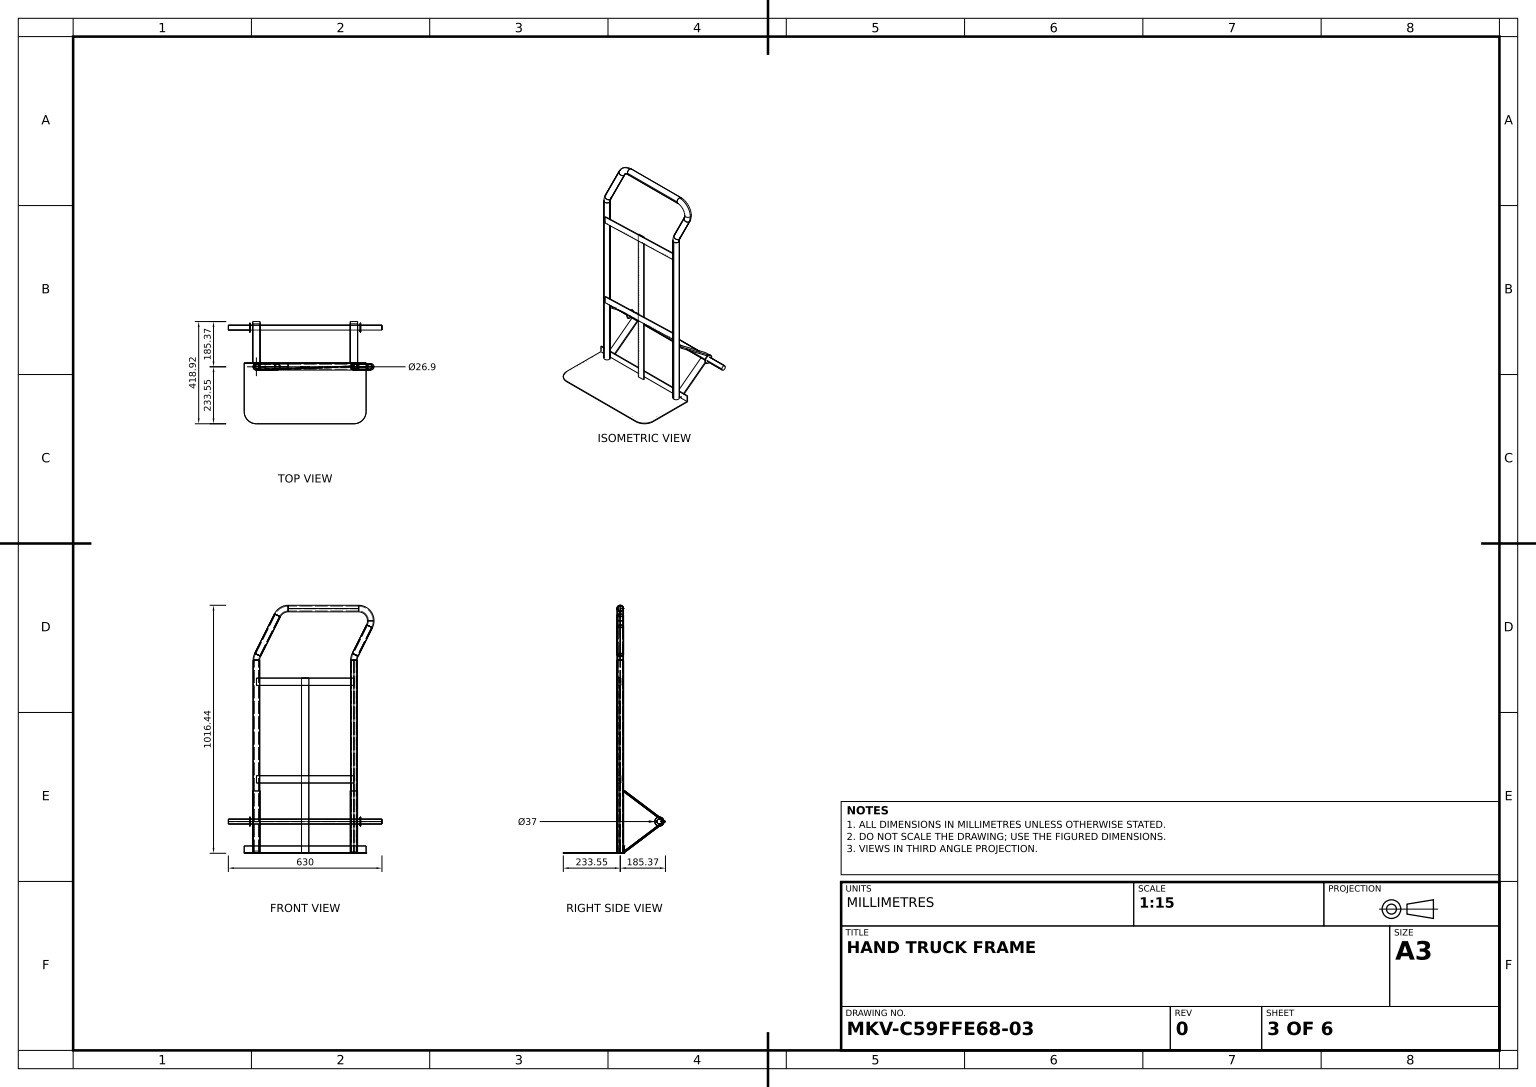
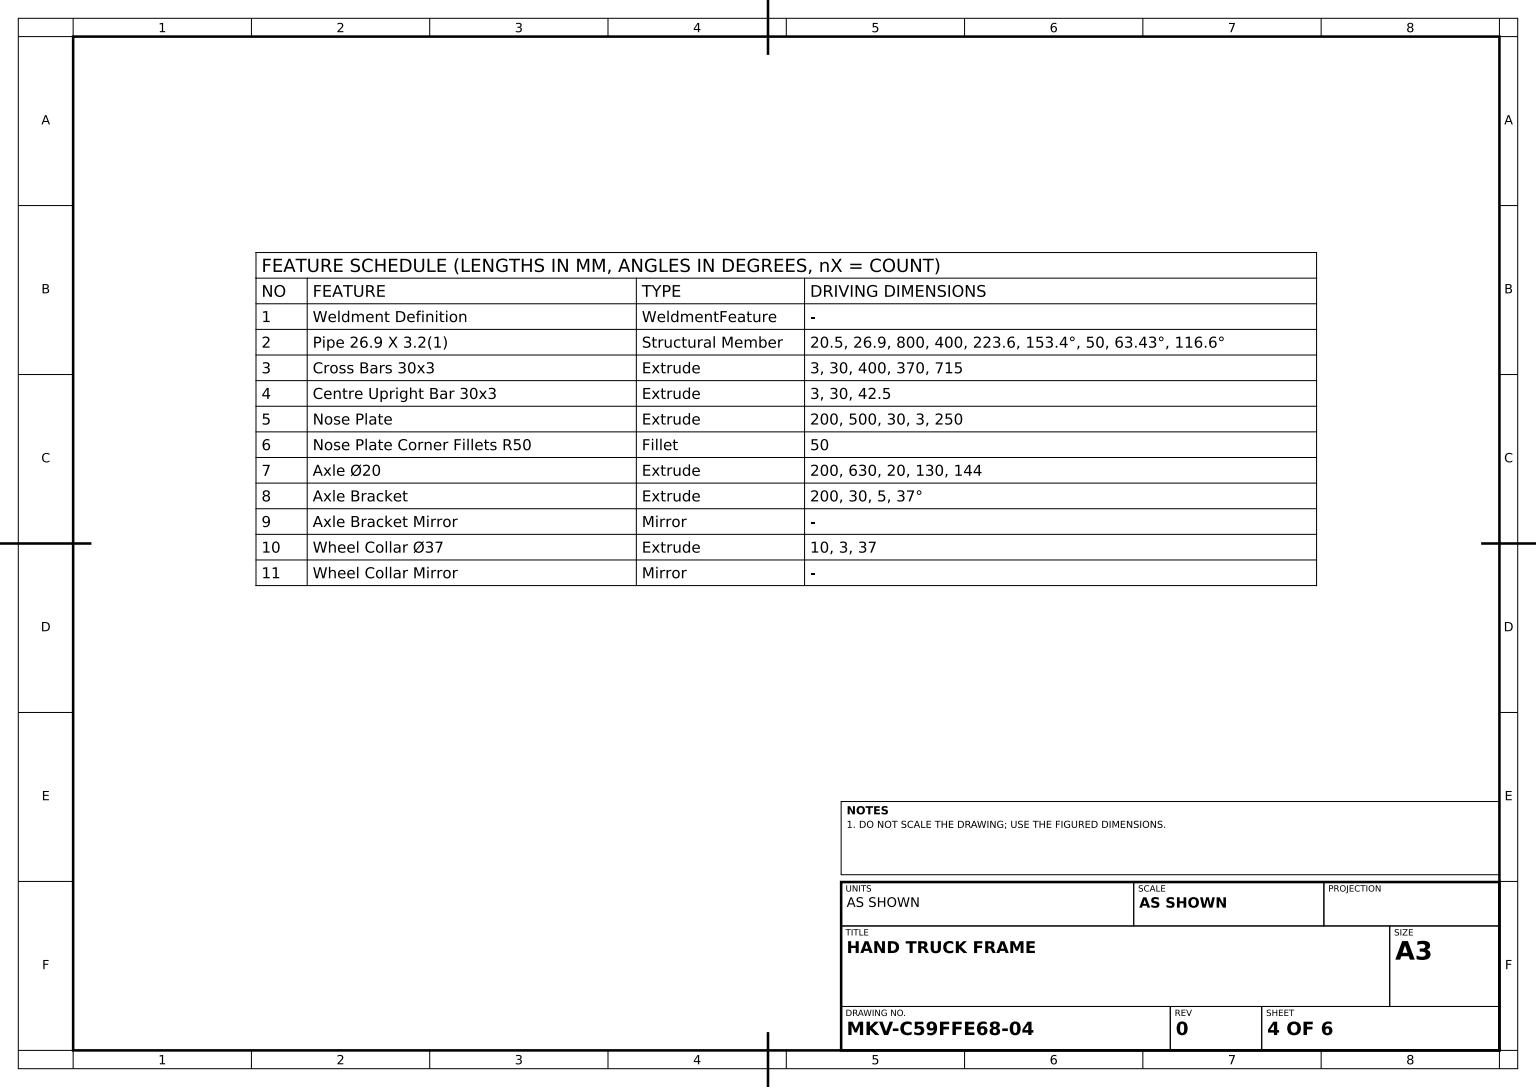
solid
v1 (-406.748954,816.574926,0)
v2 (-413.45,788.194321,0)
e1 v1 v2 CIRCLE(AX(P(-350,788.194321,0),D(0,0,1),D(0,-1,0)),63.45)
v3 (-382.689902,804.542802,0)
e2 v1 v3 CIRCLE(AX(P(-394.719428,810.558864,0),D(-0.447290848,-0.89438856,0),D(-0.89438856,0.447290848,0)),13.45)
v4 (-386.55,788.194321,0)
e3 v3 v4 CIRCLE(AX(P(-350,788.194321,0),D(0,0,1),D(0,-1,0)),36.55)
e4 v4 v2 CIRCLE(AX(P(-400,788.194321,0),D(0,1,0),D(1,0,0)),13.45)
face TORUS(AX(P(-350,788.194321,0),D(0,0,1),D(1,0,0)),50,13.45) [-e1 e2 e3 e4]
e5 v2 v4 CIRCLE(AX(P(-400,788.194321,0),D(0,1,0),D(1,0,0)),13.45)
e6 v3 v1 CIRCLE(AX(P(-394.719428,810.558864,0),D(-0.447290848,-0.89438856,0),D(-0.89438856,0.447290848,0)),13.45)
face TORUS(AX(P(-350,788.194321,0),D(0,0,1),D(1,0,0)),50,13.45) [e5 -e3 e6 e1]
v5 (-403.886911,815.143595,0)
v6 (-385.551945,805.974133,0)
e7 v5 v6 CIRCLE(AX(P(-394.719428,810.558864,0),D(0.447290848,0.89438856,0),D(-0.89438856,0.447290848,0)),10.25)
e8 v6 v5 CIRCLE(AX(P(-394.719428,810.558864,0),D(0.447290848,0.89438856,0),D(-0.89438856,0.447290848,0)),10.25)
face PLANE(AX(P(-394.719428,810.558864,0),D(0.447290848,0.89438856,0),D(-0.89438856,0.447290848,0))) [-e7 -e8] [-e2 -e6]
v7 (-389.75,788.194321,0)
e9 v6 v7 CIRCLE(AX(P(-350,788.194321,0),D(0,0,1),D(0,-1,0)),39.75)
v8 (-410.25,788.194321,0)
e10 v7 v8 CIRCLE(AX(P(-400,788.194321,0),D(0,-1,0),D(1,0,0)),10.25)
e11 v5 v8 CIRCLE(AX(P(-350,788.194321,0),D(0,0,1),D(0,-1,0)),60.25)
face TORUS(AX(P(-350,788.194321,0),D(0,0,1),D(1,0,0)),50,10.25) rev [e9 e10 -e11 e7]
e12 v8 v7 CIRCLE(AX(P(-400,788.194321,0),D(0,-1,0),D(1,0,0)),10.25)
face PLANE(AX(P(-400,788.194321,0),D(0,-1,0),D(1,0,0))) [-e4 -e5] [-e10 -e12]
face TORUS(AX(P(-350,788.194321,0),D(0,0,1),D(1,0,0)),50,10.25) rev [e8 e11 e12 -e9]
solid
v9 (0,788.194321,-13.45)
v10 (0,788.194321,13.45)
e13 v9 v10 CIRCLE(AX(P(0,788.194321,0),D(0,1,0),D(0,0,1)),13.45)
e14 v10 v9 CIRCLE(AX(P(0,788.194321,0),D(0,1,0),D(0,0,1)),13.45)
v11 (0,788.194321,10.25)
v12 (0,788.194321,-10.25)
e15 v11 v12 CIRCLE(AX(P(0,788.194321,0),D(0,1,0),D(0,0,1)),10.25)
e16 v12 v11 CIRCLE(AX(P(0,788.194321,0),D(0,1,0),D(0,0,1)),10.25)
face PLANE(AX(P(0,788.194321,0),D(0,1,0),D(0,0,1))) [e13 e14] [-e15 -e16]
v13 (0,0,10.25)
v14 (0,0,-10.25)
e17 v13 v14 CIRCLE(AX(P(0,0,0),D(0,1,0),D(0,0,1)),10.25)
e18 v11 v13 LINE
e19 v12 v14 LINE
face CYL(AX(P(0,788.194321,0),D(0,-1,0),D(0,0,-1)),10.25) rev [-e17 -e18 e15 e19]
e20 v14 v13 CIRCLE(AX(P(0,0,0),D(0,1,0),D(0,0,1)),10.25)
face CYL(AX(P(0,788.194321,0),D(0,-1,0),D(0,0,-1)),10.25) rev [-e20 -e19 e16 e18]
v15 (0,0,13.45)
v16 (0,0,-13.45)
e21 v15 v16 CIRCLE(AX(P(0,0,0),D(0,1,0),D(0,0,1)),13.45)
e22 v16 v15 CIRCLE(AX(P(0,0,0),D(0,1,0),D(0,0,1)),13.45)
face PLANE(AX(P(0,0,0),D(0,1,0),D(0,0,1))) rev [-e21 -e22] [e17 e20]
e23 v10 v15 LINE
e24 v9 v16 LINE
face CYL(AX(P(0,788.194321,0),D(0,-1,0),D(0,0,-1)),13.45) [e23 e21 -e24 -e14]
face CYL(AX(P(0,788.194321,0),D(0,-1,0),D(0,0,-1)),13.45) [e24 e22 -e23 -e13]
solid
v17 (-304.638996,967.765093,0)
v18 (-322.973962,976.934556,0)
e25 v17 v18 CIRCLE(AX(P(-313.806479,972.349825,0),D(0.447290848,0.89438856,0),D(-0.89438856,0.447290848,0)),10.25)
e26 v18 v17 CIRCLE(AX(P(-313.806479,972.349825,0),D(0.447290848,0.89438856,0),D(-0.89438856,0.447290848,0)),10.25)
v19 (-301.776953,966.333763,0)
v20 (-325.836005,978.365886,0)
e27 v19 v20 CIRCLE(AX(P(-313.806479,972.349825,0),D(0.447290848,0.89438856,0),D(-0.89438856,0.447290848,0)),13.45)
e28 v20 v19 CIRCLE(AX(P(-313.806479,972.349825,0),D(0.447290848,0.89438856,0),D(-0.89438856,0.447290848,0)),13.45)
face PLANE(AX(P(-313.806479,972.349825,0),D(0.447290848,0.89438856,0),D(-0.89438856,0.447290848,0))) [-e25 -e26] [e27 e28]
v21 (-406.748954,816.574926,0)
e29 v21 v20 LINE
v22 (-382.689902,804.542802,0)
e30 v22 v21 CIRCLE(AX(P(-394.719428,810.558864,0),D(-0.447290848,-0.89438856,0),D(0.89438856,-0.447290848,0)),13.45)
e31 v22 v19 LINE
face CYL(AX(P(-394.719428,810.558864,0),D(0.447290848,0.89438856,0),D(-0.89438856,0.447290848,0)),13.45) [-e29 -e30 e31 -e28]
v23 (-385.551945,805.974133,0)
v24 (-403.886911,815.143595,0)
e32 v23 v24 CIRCLE(AX(P(-394.719428,810.558864,0),D(-0.447290848,-0.89438856,0),D(0.89438856,-0.447290848,0)),10.25)
e33 v24 v18 LINE
e34 v23 v17 LINE
face CYL(AX(P(-394.719428,810.558864,0),D(0.447290848,0.89438856,0),D(-0.89438856,0.447290848,0)),10.25) rev [e32 e33 e26 -e34]
e35 v24 v23 CIRCLE(AX(P(-394.719428,810.558864,0),D(-0.447290848,-0.89438856,0),D(0.89438856,-0.447290848,0)),10.25)
e36 v21 v22 CIRCLE(AX(P(-394.719428,810.558864,0),D(-0.447290848,-0.89438856,0),D(0.89438856,-0.447290848,0)),13.45)
face PLANE(AX(P(-394.719428,810.558864,0),D(-0.447290848,-0.89438856,0),D(0.89438856,-0.447290848,0))) [-e35 -e32] [e36 e30]
face CYL(AX(P(-394.719428,810.558864,0),D(0.447290848,0.89438856,0),D(-0.89438856,0.447290848,0)),13.45) [-e27 -e31 -e36 e29]
face CYL(AX(P(-394.719428,810.558864,0),D(0.447290848,0.89438856,0),D(-0.89438856,0.447290848,0)),10.25) rev [-e33 e35 e34 e25]
solid
v25 (0.012157,315,-3.002106)
v26 (-399.761651,315,10.447894)
e37 v25 v26 LINE
v27 (-399.660776,315,13.446197)
e38 v26 v27 LINE
v28 (0.113032,315,-0.003803)
e39 v28 v27 LINE
e40 v25 v28 LINE
face PLANE(AX(P(0.012157,315,-3.002106),D(0,1,0),D(-1,0,0))) [e37 e38 -e39 -e40]
v29 (-399.660776,285,13.446197)
e41 v27 v29 LINE
v30 (0.113032,285,-0.003803)
e42 v29 v30 LINE
e43 v30 v28 LINE
face PLANE(AX(P(0,0,0),D(-0.033625,0,-0.99943452),D(-0.99943452,0,0.033625))) rev [e41 e42 e43 e39]
v31 (-399.761651,285,10.447894)
e44 v31 v29 LINE
v32 (0.012157,285,-3.002106)
e45 v31 v32 LINE
e46 v32 v30 LINE
face PLANE(AX(P(0.012157,285,-3.002106),D(0,-1,0),D(1,0,0))) [-e42 -e44 e45 e46]
e47 v32 v25 LINE
face PLANE(AX(P(0.012157,315,-3.002106),D(0.99943452,0,-0.033625),D(-0.033625,0,-0.99943452))) [e47 e40 -e43 -e46]
e48 v26 v31 LINE
face PLANE(AX(P(-0.100875,0,-2.998304),D(-0.033625,0,-0.99943452),D(-0.99943452,0,0.033625))) [-e45 -e48 -e37 -e47]
face PLANE(AX(P(-399.761651,315,10.447894),D(-0.99943452,0,0.033625),D(0.033625,0,0.99943452))) [-e38 e48 e44 -e41]
solid
v33 (25,127,-178.95)
v34 (25,127,-141.95)
e49 v33 v34 CIRCLE(AX(P(25,127,-160.45),D(1,0,0),D(0,0,-1)),18.5)
e50 v34 v33 CIRCLE(AX(P(25,127,-160.45),D(1,0,0),D(0,0,-1)),18.5)
face PLANE(AX(P(25,127,-160.45),D(1,0,0),D(0,0,-1))) rev [-e49 -e50]
v35 (28,127,-141.95)
v36 (28,127,-178.95)
e51 v35 v36 CIRCLE(AX(P(28,127,-160.45),D(1,0,0),D(0,0,-1)),18.5)
e52 v36 v35 CIRCLE(AX(P(28,127,-160.45),D(1,0,0),D(0,0,-1)),18.5)
face PLANE(AX(P(28,127,-160.45),D(1,0,0),D(0,0,-1))) [e51 e52]
e53 v36 v33 LINE
e54 v35 v34 LINE
face CYL(AX(P(28,127,-160.45),D(-1,0,0),D(0,0,1)),18.5) [-e53 -e51 e54 e50]
face CYL(AX(P(28,127,-160.45),D(-1,0,0),D(0,0,1)),18.5) [-e54 -e52 e53 e49]
solid
v37 (15,250.293802,-13.45)
v38 (-15,250.293802,-13.45)
e55 v37 v38 LINE
v39 (15,254.286979,-16.459075)
e56 v39 v37 LINE
v40 (-15,254.286979,-16.459075)
e57 v39 v40 LINE
e58 v40 v38 LINE
face PLANE(AX(P(15,250.293802,-13.45),D(0,-0.601815023,-0.79863551),D(0,0.79863551,-0.601815023))) rev [-e55 -e56 e57 e58]
v41 (15,127,-177.066401)
e59 v37 v41 LINE
v42 (15,3.706198,-13.45)
e60 v41 v42 LINE
v43 (15,-0.286979,-16.459075)
e61 v42 v43 LINE
v44 (15,127,-185.374602)
e62 v43 v44 LINE
e63 v44 v39 LINE
face PLANE(AX(P(15,0,0),D(1,0,0),D(0,0,-1))) [e59 e60 e61 e62 e63 e56]
v45 (-15,127,-177.066401)
e64 v38 v45 LINE
e65 v41 v45 LINE
face PLANE(AX(P(15,127,-177.066401),D(0,0.79863551,-0.601815023),D(0,0.601815023,0.79863551))) rev [-e59 e55 e64 -e65]
v46 (-15,3.706198,-13.45)
e66 v42 v46 LINE
v47 (-15,-0.286979,-16.459075)
e67 v46 v47 LINE
e68 v43 v47 LINE
face PLANE(AX(P(15,3.706198,-13.45),D(0,0.601815023,-0.79863551),D(0,0.79863551,0.601815023))) rev [-e61 e66 e67 -e68]
v48 (-15,127,-185.374602)
e69 v44 v48 LINE
e70 v48 v40 LINE
face PLANE(AX(P(15,127,-185.374602),D(0,-0.79863551,0.601815023),D(0,-0.601815023,-0.79863551))) rev [-e63 e69 e70 -e57]
e71 v45 v46 LINE
face PLANE(AX(P(15,127,-177.066401),D(0,-0.79863551,-0.601815023),D(0,0.601815023,-0.79863551))) rev [-e66 -e60 e65 e71]
e72 v47 v48 LINE
face PLANE(AX(P(15,127,-185.374602),D(0,0.79863551,0.601815023),D(0,-0.601815023,0.79863551))) rev [e68 e72 -e69 -e62]
face PLANE(AX(P(-15,0,0),D(1,0,0),D(0,0,-1))) rev [-e67 -e71 -e64 -e58 -e70 -e72]
solid
v49 (-184.984104,0,0.220215)
v50 (-214.96714,0,1.228965)
e73 v49 v50 LINE
v51 (-214.96714,715,1.228965)
e74 v50 v51 LINE
v52 (-184.984104,715,0.220215)
e75 v51 v52 LINE
e76 v52 v49 LINE
face PLANE(AX(P(-0.20175,0,-5.996607),D(0.033625,0,0.99943452),D(0.99943452,0,-0.033625))) rev [e73 e74 e75 e76]
v53 (-214.866265,0,4.227269)
e77 v50 v53 LINE
v54 (-214.866265,715,4.227269)
e78 v53 v54 LINE
e79 v51 v54 LINE
face PLANE(AX(P(-214.96714,0,1.228965),D(0.99943452,0,-0.033625),D(-0.033625,0,-0.99943452))) rev [-e74 e77 e78 -e79]
v55 (-184.883229,715,3.218519)
e80 v52 v55 LINE
e81 v54 v55 LINE
face PLANE(AX(P(-184.984104,715,0.220215),D(0,-1,0),D(0,0,-1))) rev [-e80 -e75 e79 e81]
v56 (-184.883229,0,3.218519)
e82 v55 v56 LINE
e83 v56 v53 LINE
face PLANE(AX(P(-0.100875,0,-2.998304),D(0.033625,0,0.99943452),D(0.99943452,0,-0.033625))) [-e82 -e81 -e78 -e83]
e84 v49 v56 LINE
face PLANE(AX(P(-184.984104,0,0.220215),D(0,1,0),D(0,0,1))) rev [-e77 -e73 e84 e83]
face PLANE(AX(P(-184.984104,0,0.220215),D(-0.99943452,0,0.033625),D(0.033625,0,0.99943452))) rev [-e76 e80 e82 -e84]
solid
v57 (-269.087051,989.735282,0)
v58 (-269.087051,1010.235282,0)
e85 v57 v58 CIRCLE(AX(P(-269.087051,999.985282,0),D(1,0,0),D(0,1,0)),10.25)
v59 (-322.973962,976.934556,0)
e86 v58 v59 CIRCLE(AX(P(-269.087051,949.985282,0),D(0,0,1),D(1,0,0)),60.25)
v60 (-304.638996,967.765093,0)
e87 v59 v60 CIRCLE(AX(P(-313.806479,972.349825,0),D(-0.447290848,-0.89438856,0),D(0.89438856,-0.447290848,0)),10.25)
e88 v57 v60 CIRCLE(AX(P(-269.087051,949.985282,0),D(0,0,1),D(1,0,0)),39.75)
face TORUS(AX(P(-269.087051,949.985282,0),D(0,0,1),D(1,0,0)),50,10.25) rev [e85 e86 e87 -e88]
e89 v60 v59 CIRCLE(AX(P(-313.806479,972.349825,0),D(-0.447290848,-0.89438856,0),D(0.89438856,-0.447290848,0)),10.25)
e90 v58 v57 CIRCLE(AX(P(-269.087051,999.985282,0),D(1,0,0),D(0,1,0)),10.25)
face TORUS(AX(P(-269.087051,949.985282,0),D(0,0,1),D(1,0,0)),50,10.25) rev [e89 -e86 e90 e88]
v61 (-269.087051,986.535282,0)
v62 (-301.776953,966.333763,0)
e91 v61 v62 CIRCLE(AX(P(-269.087051,949.985282,0),D(0,0,1),D(1,0,0)),36.55)
v63 (-325.836005,978.365886,0)
e92 v62 v63 CIRCLE(AX(P(-313.806479,972.349825,0),D(0.447290848,0.89438856,0),D(0.89438856,-0.447290848,0)),13.45)
v64 (-269.087051,1013.435282,0)
e93 v64 v63 CIRCLE(AX(P(-269.087051,949.985282,0),D(0,0,1),D(1,0,0)),63.45)
e94 v64 v61 CIRCLE(AX(P(-269.087051,999.985282,0),D(-1,0,0),D(0,1,0)),13.45)
face TORUS(AX(P(-269.087051,949.985282,0),D(0,0,1),D(1,0,0)),50,13.45) [e91 e92 -e93 e94]
e95 v61 v64 CIRCLE(AX(P(-269.087051,999.985282,0),D(-1,0,0),D(0,1,0)),13.45)
face PLANE(AX(P(-269.087051,999.985282,0),D(1,0,0),D(0,1,0))) [-e95 -e94] [-e90 -e85]
e96 v63 v62 CIRCLE(AX(P(-313.806479,972.349825,0),D(0.447290848,0.89438856,0),D(0.89438856,-0.447290848,0)),13.45)
face PLANE(AX(P(-313.806479,972.349825,0),D(-0.447290848,-0.89438856,0),D(0.89438856,-0.447290848,0))) [-e96 -e92] [-e87 -e89]
face TORUS(AX(P(-269.087051,949.985282,0),D(0,0,1),D(1,0,0)),50,13.45) [-e91 e95 e93 e96]
solid
v65 (51.794623,933.636802,0)
v66 (-6.748954,816.574926,0)
e97 v65 v66 LINE
v67 (17.310098,804.542802,0)
e98 v67 v66 CIRCLE(AX(P(5.280572,810.558864,0),D(-0.447290848,-0.89438856,0),D(0.89438856,-0.447290848,0)),13.45)
v68 (75.853675,921.604678,0)
e99 v68 v67 LINE
e100 v65 v68 CIRCLE(AX(P(63.824149,927.62074,0),D(0.447290848,0.89438856,0),D(-0.89438856,0.447290848,0)),13.45)
face CYL(AX(P(63.824149,927.62074,0),D(-0.447290848,-0.89438856,0),D(0.89438856,-0.447290848,0)),13.45) [e97 -e98 -e99 -e100]
e101 v66 v67 CIRCLE(AX(P(5.280572,810.558864,0),D(-0.447290848,-0.89438856,0),D(0.89438856,-0.447290848,0)),13.45)
v69 (14.448055,805.974133,0)
v70 (-3.886911,815.143595,0)
e102 v69 v70 CIRCLE(AX(P(5.280572,810.558864,0),D(-0.447290848,-0.89438856,0),D(0.89438856,-0.447290848,0)),10.25)
e103 v70 v69 CIRCLE(AX(P(5.280572,810.558864,0),D(-0.447290848,-0.89438856,0),D(0.89438856,-0.447290848,0)),10.25)
face PLANE(AX(P(5.280572,810.558864,0),D(-0.447290848,-0.89438856,0),D(0.89438856,-0.447290848,0))) [e101 e98] [-e102 -e103]
v71 (72.991632,923.036008,0)
e104 v71 v69 LINE
v72 (54.656666,932.205471,0)
e105 v71 v72 CIRCLE(AX(P(63.824149,927.62074,0),D(0.447290848,0.89438856,0),D(-0.89438856,0.447290848,0)),10.25)
e106 v72 v70 LINE
face CYL(AX(P(63.824149,927.62074,0),D(-0.447290848,-0.89438856,0),D(0.89438856,-0.447290848,0)),10.25) rev [e103 -e104 e105 e106]
e107 v68 v65 CIRCLE(AX(P(63.824149,927.62074,0),D(0.447290848,0.89438856,0),D(-0.89438856,0.447290848,0)),13.45)
e108 v72 v71 CIRCLE(AX(P(63.824149,927.62074,0),D(0.447290848,0.89438856,0),D(-0.89438856,0.447290848,0)),10.25)
face PLANE(AX(P(63.824149,927.62074,0),D(0.447290848,0.89438856,0),D(-0.89438856,0.447290848,0))) [e100 e107] [-e108 -e105]
face CYL(AX(P(63.824149,927.62074,0),D(-0.447290848,-0.89438856,0),D(0.89438856,-0.447290848,0)),10.25) rev [-e106 e108 e104 e102]
face CYL(AX(P(63.824149,927.62074,0),D(-0.447290848,-0.89438856,0),D(0.89438856,-0.447290848,0)),13.45) [-e107 e99 -e101 -e97]
solid
v73 (-413.45,0,0)
v74 (-386.55,0,0)
e109 v73 v74 CIRCLE(AX(P(-400,0,0),D(0,-1,0),D(0,0,1)),13.45)
e110 v74 v73 CIRCLE(AX(P(-400,0,0),D(0,-1,0),D(0,0,1)),13.45)
v75 (-389.75,0,0)
v76 (-410.25,0,0)
e111 v75 v76 CIRCLE(AX(P(-400,0,0),D(0,-1,0),D(0,0,1)),10.25)
e112 v76 v75 CIRCLE(AX(P(-400,0,0),D(0,-1,0),D(0,0,1)),10.25)
face PLANE(AX(P(-400,0,0),D(0,-1,0),D(0,0,1))) [e109 e110] [-e111 -e112]
v77 (-386.55,788.194321,0)
v78 (-413.45,788.194321,0)
e113 v77 v78 CIRCLE(AX(P(-400,788.194321,0),D(0,1,0),D(-1,0,0)),13.45)
e114 v78 v77 CIRCLE(AX(P(-400,788.194321,0),D(0,1,0),D(-1,0,0)),13.45)
v79 (-389.75,788.194321,0)
v80 (-410.25,788.194321,0)
e115 v79 v80 CIRCLE(AX(P(-400,788.194321,0),D(0,1,0),D(-1,0,0)),10.25)
e116 v80 v79 CIRCLE(AX(P(-400,788.194321,0),D(0,1,0),D(-1,0,0)),10.25)
face PLANE(AX(P(-400,788.194321,0),D(0,1,0),D(-1,0,0))) [e113 e114] [-e115 -e116]
e117 v76 v80 LINE
e118 v75 v79 LINE
face CYL(AX(P(-400,0,0),D(0,1,0),D(-1,0,0)),10.25) rev [e117 e116 -e118 e111]
e119 v73 v78 LINE
e120 v74 v77 LINE
face CYL(AX(P(-400,0,0),D(0,1,0),D(-1,0,0)),13.45) [-e114 -e119 -e110 e120]
face CYL(AX(P(-400,0,0),D(0,1,0),D(-1,0,0)),10.25) rev [e118 e115 -e117 e112]
face CYL(AX(P(-400,0,0),D(0,1,0),D(-1,0,0)),13.45) [-e109 e119 -e113 -e120]
solid
v81 (-269.087051,999.985282,10.25)
v82 (19.104721,999.985282,10.25)
e121 v81 v82 LINE
v83 (-269.087051,999.985282,-10.25)
e122 v81 v83 CIRCLE(AX(P(-269.087051,999.985282,0),D(-1,0,0),D(0,-1,0)),10.25)
v84 (19.104721,999.985282,-10.25)
e123 v83 v84 LINE
e124 v84 v82 CIRCLE(AX(P(19.104721,999.985282,0),D(1,0,0),D(0,1,0)),10.25)
face CYL(AX(P(-269.087051,999.985282,0),D(1,0,0),D(0,0,-1)),10.25) rev [-e121 e122 e123 e124]
v85 (-269.087051,999.985282,-13.45)
v86 (19.104721,999.985282,-13.45)
e125 v85 v86 LINE
v87 (-269.087051,999.985282,13.45)
e126 v87 v85 CIRCLE(AX(P(-269.087051,999.985282,0),D(-1,0,0),D(0,-1,0)),13.45)
v88 (19.104721,999.985282,13.45)
e127 v87 v88 LINE
e128 v86 v88 CIRCLE(AX(P(19.104721,999.985282,0),D(1,0,0),D(0,1,0)),13.45)
face CYL(AX(P(-269.087051,999.985282,0),D(1,0,0),D(0,0,-1)),13.45) [-e125 -e126 e127 -e128]
e129 v88 v86 CIRCLE(AX(P(19.104721,999.985282,0),D(1,0,0),D(0,1,0)),13.45)
e130 v82 v84 CIRCLE(AX(P(19.104721,999.985282,0),D(1,0,0),D(0,1,0)),10.25)
face PLANE(AX(P(19.104721,999.985282,0),D(1,0,0),D(0,1,0))) [e128 e129] [-e124 -e130]
e131 v85 v87 CIRCLE(AX(P(-269.087051,999.985282,0),D(-1,0,0),D(0,-1,0)),13.45)
face CYL(AX(P(-269.087051,999.985282,0),D(1,0,0),D(0,0,-1)),13.45) [-e129 -e127 -e131 e125]
e132 v83 v81 CIRCLE(AX(P(-269.087051,999.985282,0),D(-1,0,0),D(0,-1,0)),10.25)
face CYL(AX(P(-269.087051,999.985282,0),D(1,0,0),D(0,0,-1)),10.25) rev [e132 e121 e130 -e123]
face PLANE(AX(P(-269.087051,999.985282,0),D(-1,0,0),D(0,-1,0))) [e126 e131] [-e122 -e132]
solid
v89 (-425,127,-170.45)
v90 (-425,127,-150.45)
e133 v89 v90 CIRCLE(AX(P(-425,127,-160.45),D(-1,0,0),D(0,0,1)),10)
e134 v90 v89 CIRCLE(AX(P(-425,127,-160.45),D(-1,0,0),D(0,0,1)),10)
v91 (-425,127,-141.95)
v92 (-425,127,-178.95)
e135 v91 v92 CIRCLE(AX(P(-425,127,-160.45),D(1,0,0),D(0,0,-1)),18.5)
e136 v92 v91 CIRCLE(AX(P(-425,127,-160.45),D(1,0,0),D(0,0,-1)),18.5)
face PLANE(AX(P(-425,127,-160.45),D(-1,0,0),D(0,0,-1))) rev [e133 e134] [e135 e136]
v93 (-428,127,-150.45)
v94 (-428,127,-170.45)
e137 v93 v94 CIRCLE(AX(P(-428,127,-160.45),D(-1,0,0),D(0,0,1)),10)
v95 (-515,127,-170.45)
e138 v94 v95 LINE
v96 (-515,127,-150.45)
e139 v95 v96 CIRCLE(AX(P(-515,127,-160.45),D(1,0,0),D(0,0,-1)),10)
e140 v93 v96 LINE
face CYL(AX(P(115,127,-160.45),D(-1,0,0),D(0,0,1)),10) [e137 e138 e139 -e140]
v97 (115,127,-150.45)
v98 (115,127,-170.45)
e141 v97 v98 CIRCLE(AX(P(115,127,-160.45),D(1,0,0),D(0,0,-1)),10)
e142 v98 v97 CIRCLE(AX(P(115,127,-160.45),D(1,0,0),D(0,0,-1)),10)
face PLANE(AX(P(115,127,-160.45),D(1,0,0),D(0,0,-1))) [e141 e142]
e143 v96 v95 CIRCLE(AX(P(-515,127,-160.45),D(1,0,0),D(0,0,-1)),10)
e144 v94 v93 CIRCLE(AX(P(-428,127,-160.45),D(-1,0,0),D(0,0,1)),10)
face CYL(AX(P(115,127,-160.45),D(-1,0,0),D(0,0,1)),10) [e140 e143 -e138 e144]
e145 v97 v90 LINE
e146 v98 v89 LINE
face CYL(AX(P(115,127,-160.45),D(-1,0,0),D(0,0,1)),10) [-e145 -e142 e146 -e134]
v99 (-428,127,-178.95)
e147 v99 v92 LINE
v100 (-428,127,-141.95)
e148 v99 v100 CIRCLE(AX(P(-428,127,-160.45),D(1,0,0),D(0,0,-1)),18.5)
e149 v100 v91 LINE
face CYL(AX(P(-428,127,-160.45),D(1,0,0),D(0,0,1)),18.5) [-e136 -e147 e148 e149]
face PLANE(AX(P(-515,127,-160.45),D(1,0,0),D(0,0,-1))) rev [-e139 -e143]
e150 v100 v99 CIRCLE(AX(P(-428,127,-160.45),D(1,0,0),D(0,0,-1)),18.5)
face PLANE(AX(P(-428,127,-160.45),D(-1,0,0),D(0,0,-1))) [-e148 -e150] [-e144 -e137]
face CYL(AX(P(-428,127,-160.45),D(1,0,0),D(0,0,1)),18.5) [e150 e147 -e135 -e149]
face CYL(AX(P(115,127,-160.45),D(-1,0,0),D(0,0,1)),10) [-e133 -e146 -e141 e145]
solid
v101 (-415,254.286979,-16.459075)
v102 (-415,250.293802,-13.45)
e151 v101 v102 LINE
v103 (-385,250.293802,-13.45)
e152 v102 v103 LINE
v104 (-385,254.286979,-16.459075)
e153 v104 v103 LINE
e154 v101 v104 LINE
face PLANE(AX(P(-415,250.293802,-13.45),D(0,-0.601815023,-0.79863551),D(0,0.79863551,-0.601815023))) rev [e151 e152 -e153 -e154]
v105 (-450,-3,183.55)
v106 (-450,0,183.55)
e155 v105 v106 LINE
v107 (-400,-3,233.55)
e156 v107 v105 CIRCLE(AX(P(-400,-3,183.55),D(0,-1,0),D(0,0,1)),50)
v108 (-400,0,233.55)
e157 v108 v107 LINE
e158 v106 v108 CIRCLE(AX(P(-400,0,183.55),D(0,1,0),D(0,0,-1)),50)
face CYL(AX(P(-400,0,183.55),D(0,1,0),D(0,0,1)),50) [-e155 -e156 -e157 -e158]
v109 (-450,27,-16.45)
v110 (-450,27,-13.45)
e159 v109 v110 LINE
v111 (50,27,-13.45)
e160 v111 v110 LINE
v112 (50,27,-16.45)
e161 v112 v111 LINE
e162 v112 v109 LINE
face PLANE(AX(P(50,27,-13.45),D(0,-1,0),D(0,0,-1))) rev [e159 -e160 -e161 e162]
v113 (-415,-0.286979,-16.459075)
v114 (-385,-0.286979,-16.459075)
e163 v113 v114 LINE
v115 (-385,-0.274936,-16.45)
e164 v115 v114 LINE
v116 (-415,-0.274936,-16.45)
e165 v115 v116 LINE
e166 v116 v113 LINE
face PLANE(AX(P(-415,3.706198,-13.45),D(0,0.601815023,-0.79863551),D(0,0.79863551,0.601815023))) rev [e163 -e164 e165 e166]
v117 (-415,127,-177.066401)
e167 v102 v117 LINE
v118 (-385,127,-177.066401)
e168 v117 v118 LINE
e169 v103 v118 LINE
face PLANE(AX(P(-415,127,-177.066401),D(0,0.79863551,-0.601815023),D(0,0.601815023,0.79863551))) rev [-e152 e167 e168 -e169]
v119 (-450,-3,-16.45)
e170 v105 v119 LINE
v120 (50,-3,-16.45)
e171 v120 v119 LINE
v121 (50,-3,183.55)
e172 v121 v120 LINE
v122 (0,-3,233.55)
e173 v121 v122 CIRCLE(AX(P(0,-3,183.55),D(0,-1,0),D(0,0,1)),50)
e174 v122 v107 LINE
face PLANE(AX(P(50,-3,-16.45),D(0,1,0),D(0,0,1))) rev [e156 e170 -e171 -e172 e173 e174]
e175 v119 v109 LINE
e176 v120 v112 LINE
v123 (-415,5.96686,-16.45)
v124 (-385,5.96686,-16.45)
e177 v123 v124 LINE
e178 v123 v116 LINE
e179 v124 v115 LINE
face PLANE(AX(P(50,27,-16.45),D(0,0,1),D(0,-1,0))) rev [e175 -e162 -e176 e171] [-e177 e178 -e165 -e179]
v125 (-415,127,-185.374602)
e180 v125 v101 LINE
v126 (-385,127,-185.374602)
e181 v126 v104 LINE
e182 v125 v126 LINE
face PLANE(AX(P(-415,127,-185.374602),D(0,-0.79863551,0.601815023),D(0,-0.601815023,-0.79863551))) rev [e180 e154 -e181 -e182]
e183 v114 v126 LINE
e184 v118 v124 LINE
face PLANE(AX(P(-385,0,0),D(-1,0,0),D(0,0,-1))) rev [e164 e183 e181 e153 e169 e184 e179]
e185 v117 v123 LINE
face PLANE(AX(P(-415,127,-177.066401),D(0,-0.79863551,-0.601815023),D(0,0.601815023,-0.79863551))) rev [-e184 -e168 e185 e177]
v127 (-450,0,-13.45)
e186 v110 v127 LINE
v128 (50,0,-13.45)
e187 v128 v127 LINE
e188 v111 v128 LINE
face PLANE(AX(P(50,27,-13.45),D(0,0,-1),D(0,1,0))) rev [e186 -e187 -e188 e160]
e189 v113 v125 LINE
face PLANE(AX(P(-415,0,0),D(-1,0,0),D(0,0,-1))) [-e189 -e166 -e178 -e185 -e167 -e151 -e180]
v129 (50,0,183.55)
e190 v129 v121 LINE
v130 (0,0,233.55)
e191 v130 v129 CIRCLE(AX(P(0,0,183.55),D(0,1,0),D(0,0,-1)),50)
e192 v122 v130 LINE
face CYL(AX(P(0,0,183.55),D(0,-1,0),D(0,0,-1)),50) [-e173 -e190 -e191 -e192]
e193 v127 v106 LINE
face PLANE(AX(P(-450,0,0),D(-1,0,0),D(0,0,1))) [-e175 -e170 e155 -e193 -e186 -e159]
e194 v130 v108 LINE
face PLANE(AX(P(50,0,233.55),D(0,0,-1),D(-1,0,0))) rev [-e174 e192 e194 e157]
e195 v128 v129 LINE
face PLANE(AX(P(50,0,-13.45),D(0,-1,0),D(0,0,-1))) rev [e191 -e195 e187 e193 e158 -e194]
face PLANE(AX(P(-415,127,-185.374602),D(0,0.79863551,0.601815023),D(0,-0.601815023,0.79863551))) rev [-e183 -e163 e189 e182]
face PLANE(AX(P(50,0,0),D(-1,0,0),D(0,0,1))) rev [e190 e172 e176 e161 e188 e195]
solid
v131 (-6.748954,816.574926,0)
v132 (17.310098,804.542802,0)
e196 v131 v132 CIRCLE(AX(P(5.280572,810.558864,0),D(-0.447290848,-0.89438856,0),D(-0.89438856,0.447290848,0)),13.45)
v133 (13.45,788.194321,0)
e197 v133 v132 CIRCLE(AX(P(50,788.194321,0),D(0,0,-1),D(-1,0,0)),36.55)
v134 (-13.45,788.194321,0)
e198 v133 v134 CIRCLE(AX(P(0,788.194321,0),D(0,1,0),D(0,0,-1)),13.45)
e199 v134 v131 CIRCLE(AX(P(50,788.194321,0),D(0,0,-1),D(-1,0,0)),63.45)
face TORUS(AX(P(50,788.194321,0),D(0,0,-1),D(-1,0,0)),50,13.45) [e196 -e197 e198 e199]
v135 (10.25,788.194321,0)
v136 (-10.25,788.194321,0)
e200 v135 v136 CIRCLE(AX(P(0,788.194321,0),D(0,-1,0),D(0,0,-1)),10.25)
v137 (-3.886911,815.143595,0)
e201 v136 v137 CIRCLE(AX(P(50,788.194321,0),D(0,0,-1),D(-1,0,0)),60.25)
v138 (14.448055,805.974133,0)
e202 v137 v138 CIRCLE(AX(P(5.280572,810.558864,0),D(0.447290848,0.89438856,0),D(-0.89438856,0.447290848,0)),10.25)
e203 v135 v138 CIRCLE(AX(P(50,788.194321,0),D(0,0,-1),D(-1,0,0)),39.75)
face TORUS(AX(P(50,788.194321,0),D(0,0,-1),D(-1,0,0)),50,10.25) rev [e200 e201 e202 -e203]
e204 v136 v135 CIRCLE(AX(P(0,788.194321,0),D(0,-1,0),D(0,0,-1)),10.25)
e205 v134 v133 CIRCLE(AX(P(0,788.194321,0),D(0,1,0),D(0,0,-1)),13.45)
face PLANE(AX(P(0,788.194321,0),D(0,-1,0),D(0,0,-1))) [-e200 -e204] [-e205 -e198]
e206 v138 v137 CIRCLE(AX(P(5.280572,810.558864,0),D(0.447290848,0.89438856,0),D(-0.89438856,0.447290848,0)),10.25)
face TORUS(AX(P(50,788.194321,0),D(0,0,-1),D(-1,0,0)),50,10.25) rev [e206 -e201 e204 e203]
e207 v132 v131 CIRCLE(AX(P(5.280572,810.558864,0),D(-0.447290848,-0.89438856,0),D(-0.89438856,0.447290848,0)),13.45)
face PLANE(AX(P(5.280572,810.558864,0),D(0.447290848,0.89438856,0),D(-0.89438856,0.447290848,0))) [-e206 -e202] [-e196 -e207]
face TORUS(AX(P(50,788.194321,0),D(0,0,-1),D(-1,0,0)),50,13.45) [e207 -e199 e205 e197]
solid
v139 (0.113032,685,-0.003803)
v140 (0.113032,715,-0.003803)
e208 v139 v140 LINE
v141 (-399.660776,715,13.446197)
e209 v140 v141 LINE
v142 (-399.660776,685,13.446197)
e210 v141 v142 LINE
e211 v142 v139 LINE
face PLANE(AX(P(0,0,0),D(-0.033625,0,-0.99943452),D(-0.99943452,0,0.033625))) rev [e208 e209 e210 e211]
v143 (0.012157,685,-3.002106)
v144 (0.012157,715,-3.002106)
e212 v143 v144 LINE
v145 (-399.761651,685,10.447894)
e213 v145 v143 LINE
v146 (-399.761651,715,10.447894)
e214 v146 v145 LINE
e215 v144 v146 LINE
face PLANE(AX(P(-0.100875,0,-2.998304),D(-0.033625,0,-0.99943452),D(-0.99943452,0,0.033625))) [-e212 -e213 -e214 -e215]
e216 v144 v140 LINE
e217 v143 v139 LINE
face PLANE(AX(P(0.012157,715,-3.002106),D(0.99943452,0,-0.033625),D(-0.033625,0,-0.99943452))) [e212 e216 -e208 -e217]
e218 v146 v141 LINE
face PLANE(AX(P(0.012157,715,-3.002106),D(0,1,0),D(-1,0,0))) [-e216 e215 e218 -e209]
e219 v145 v142 LINE
face PLANE(AX(P(-399.761651,715,10.447894),D(-0.99943452,0,0.033625),D(0.033625,0,0.99943452))) [e214 e219 -e210 -e218]
face PLANE(AX(P(0.012157,685,-3.002106),D(0,-1,0),D(1,0,0))) [e217 -e211 -e219 e213]
solid
v147 (55.654721,949.985282,0)
v148 (82.554721,949.985282,0)
e220 v147 v148 CIRCLE(AX(P(69.104721,949.985282,0),D(0,-1,0),D(0,0,-1)),13.45)
v149 (75.853675,921.604678,0)
e221 v149 v148 CIRCLE(AX(P(19.104721,949.985282,0),D(0,0,1),D(1,0,0)),63.45)
v150 (51.794623,933.636802,0)
e222 v149 v150 CIRCLE(AX(P(63.824149,927.62074,0),D(0.447290848,0.89438856,0),D(0.89438856,-0.447290848,0)),13.45)
e223 v150 v147 CIRCLE(AX(P(19.104721,949.985282,0),D(0,0,1),D(1,0,0)),36.55)
face TORUS(AX(P(19.104721,949.985282,0),D(0,0,1),D(1,0,0)),50,13.45) [e220 -e221 e222 e223]
v151 (19.104721,1013.435282,0)
v152 (19.104721,986.535282,0)
e224 v151 v152 CIRCLE(AX(P(19.104721,999.985282,0),D(1,0,0),D(0,-1,0)),13.45)
e225 v152 v151 CIRCLE(AX(P(19.104721,999.985282,0),D(1,0,0),D(0,-1,0)),13.45)
v153 (19.104721,1010.235282,0)
v154 (19.104721,989.735282,0)
e226 v153 v154 CIRCLE(AX(P(19.104721,999.985282,0),D(-1,0,0),D(0,-1,0)),10.25)
e227 v154 v153 CIRCLE(AX(P(19.104721,999.985282,0),D(-1,0,0),D(0,-1,0)),10.25)
face PLANE(AX(P(19.104721,999.985282,0),D(-1,0,0),D(0,-1,0))) [-e224 -e225] [-e226 -e227]
v155 (79.354721,949.985282,0)
e228 v155 v153 CIRCLE(AX(P(19.104721,949.985282,0),D(0,0,1),D(1,0,0)),60.25)
v156 (58.854721,949.985282,0)
e229 v155 v156 CIRCLE(AX(P(69.104721,949.985282,0),D(0,-1,0),D(0,0,-1)),10.25)
e230 v156 v154 CIRCLE(AX(P(19.104721,949.985282,0),D(0,0,1),D(1,0,0)),39.75)
face TORUS(AX(P(19.104721,949.985282,0),D(0,0,1),D(1,0,0)),50,10.25) rev [e227 -e228 e229 e230]
v157 (72.991632,923.036008,0)
v158 (54.656666,932.205471,0)
e231 v157 v158 CIRCLE(AX(P(63.824149,927.62074,0),D(-0.447290848,-0.89438856,0),D(0.89438856,-0.447290848,0)),10.25)
e232 v158 v156 CIRCLE(AX(P(19.104721,949.985282,0),D(0,0,1),D(1,0,0)),39.75)
e233 v157 v155 CIRCLE(AX(P(19.104721,949.985282,0),D(0,0,1),D(1,0,0)),60.25)
face TORUS(AX(P(19.104721,949.985282,0),D(0,0,1),D(1,0,0)),50,10.25) rev [e231 e232 -e229 -e233]
e234 v156 v155 CIRCLE(AX(P(69.104721,949.985282,0),D(0,-1,0),D(0,0,-1)),10.25)
face TORUS(AX(P(19.104721,949.985282,0),D(0,0,1),D(1,0,0)),50,10.25) rev [-e230 e234 e228 e226]
e235 v150 v149 CIRCLE(AX(P(63.824149,927.62074,0),D(0.447290848,0.89438856,0),D(0.89438856,-0.447290848,0)),13.45)
e236 v148 v147 CIRCLE(AX(P(69.104721,949.985282,0),D(0,-1,0),D(0,0,-1)),13.45)
face TORUS(AX(P(19.104721,949.985282,0),D(0,0,1),D(1,0,0)),50,13.45) [-e223 e235 e221 e236]
e237 v158 v157 CIRCLE(AX(P(63.824149,927.62074,0),D(-0.447290848,-0.89438856,0),D(0.89438856,-0.447290848,0)),10.25)
face PLANE(AX(P(63.824149,927.62074,0),D(-0.447290848,-0.89438856,0),D(0.89438856,-0.447290848,0))) [-e235 -e222] [-e237 -e231]
e238 v147 v152 CIRCLE(AX(P(19.104721,949.985282,0),D(0,0,1),D(1,0,0)),36.55)
e239 v148 v151 CIRCLE(AX(P(19.104721,949.985282,0),D(0,0,1),D(1,0,0)),63.45)
face TORUS(AX(P(19.104721,949.985282,0),D(0,0,1),D(1,0,0)),50,13.45) [-e238 -e236 e239 e224]
face TORUS(AX(P(19.104721,949.985282,0),D(0,0,1),D(1,0,0)),50,13.45) [-e220 e238 e225 -e239]
face TORUS(AX(P(19.104721,949.985282,0),D(0,0,1),D(1,0,0)),50,10.25) rev [e233 -e234 -e232 e237]
